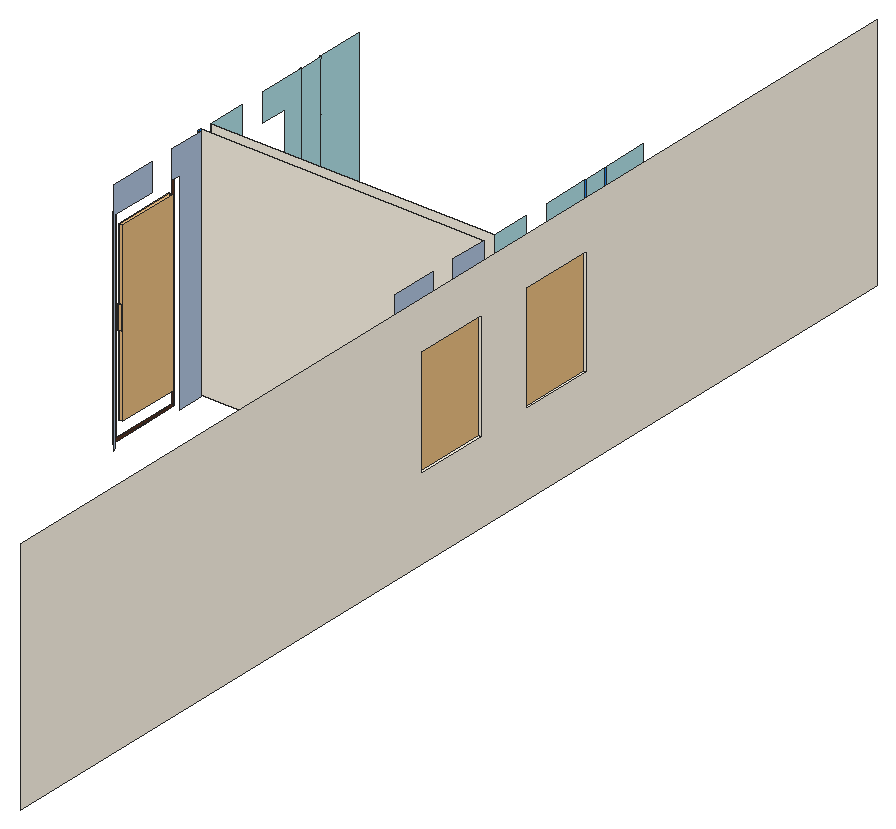
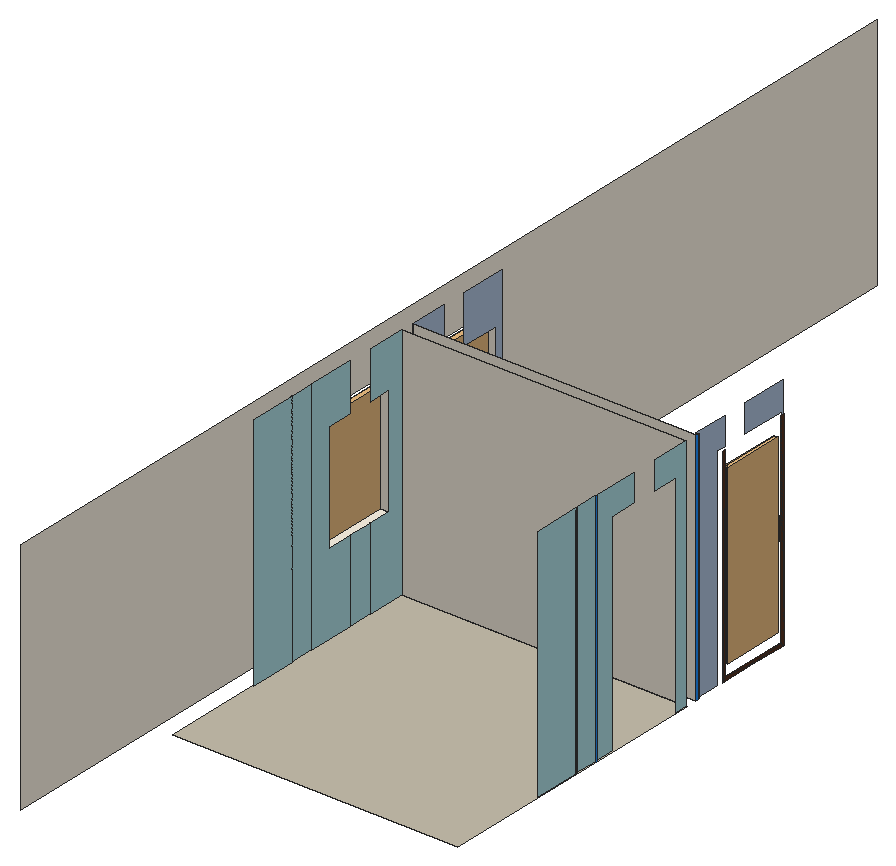
# SketchUp Ruby script. Lengths in inches.
U = 1.inch
M = Sketchup.active_model
def pt(a) = Geom::Point3d.new(a.map { |v| v * U })
def face(e, loops, mat)
  f = e.add_face(loops[0].map { |a| pt(a) })
  loops[1..].each { |l| e.add_face(l.map { |a| pt(a) }).erase! }
  f.material = f.back_material = mat if mat
  f
end
# faces: each face lists its corners as indices into pts; further lists are holes
def faces(e, pts, list, mat = nil) = list.each { |f| face(e, (f[0].is_a?(Array) ? f : [f]).map { |l| l.map { |i| pts[i] } }, mat) }
# xy, xz, yz: faces in a plane at the given z, y or x. An outline is a flat list of corners, or four numbers for a rectangle; further outlines are holes
def ring(l) = l.size == 4 ? [[l[0], l[1]], [l[2], l[1]], [l[2], l[3]], [l[0], l[3]]] : l.each_slice(2).to_a
def flat(e, list, mat, &to3) = list.each { |f| face(e, (f[0].is_a?(Array) ? f : [f]).map { |l| ring(l).map { |u, v| to3.(u, v) } }, mat) }
def xy(e, z, list, mat = nil) = flat(e, list, mat) { |x, y| [x, y, z] }
def xz(e, y, list, mat = nil) = flat(e, list, mat) { |x, z| [x, y, z] }
def yz(e, x, list, mat = nil) = flat(e, list, mat) { |y, z| [x, y, z] }
def lines(e, pts, list) = list.each { |a, b| e.add_line(pt(pts[a]), pt(pts[b])) }
# prism: a flat outline (further loops are holes) pulled along v
def prism(e, loops, v, mat = nil)
  f = face(e, loops, mat); d = Geom::Vector3d.new(v.map { |x| x * U })
  f.pushpull(f.normal.samedirection?(d) ? d.length : -d.length)
end
def box(e, o, s, mat = nil) = prism(e, [[o, [o[0] + s[0], o[1], o[2]], [o[0] + s[0], o[1] + s[1], o[2]], [o[0], o[1] + s[1], o[2]]]], [0, 0, s[2]], mat)
def at(x, y, z, deg = 0) = Geom::Transformation.translation(pt([x, y, z])) * Geom::Transformation.rotation(ORIGIN, Z_AXIS, deg.degrees)
def axes(o, x, y, z) = Geom::Transformation.new([*x, 0, *y, 0, *z, 0, *pt(o).to_a, 1])
def part(name) = M.definitions.add(name)
# library, detail: a bought-in or finely detailed component or shape, given as its bounding box
def library(name, o, s) = part(name).tap { |d| box(d.entities, o, s) }
def detail(e, o, s) = box(e.add_group.entities, o, s)
def put(e, d, t, mat = nil) = e.add_instance(d, t).tap { |i| i.material = mat if mat }
def group(e, t, mat = nil) = e.add_group.tap { |g| g.transformation = t; g.material = mat if mat }.entities
root = M.entities
M.materials.add("Material \#0").color = [86, 53, 35]
M.materials.add("Material \#1").color = [140, 140, 140]
M.materials.add("[0030_OldLace]").color = [253, 245, 230]
M.materials.add("[0094_PowderBlue]").color = [176, 224, 230]
M.materials.add("[0098_DodgerBlue]").color = [30, 144, 255]
M.materials.add("[0099_LightSteelBlue]").color = [176, 196, 222]
M.materials.add("[Tile Canvas]").color = [199, 192, 173]
c1 = library("3DGeom~4_Defintion",[-18.02,-499.97,-221.16],[36.04,1000,262.12])
c2 = part("3DGeom~5_Defintion")
xy(c2.entities,-225.24,[[-0.79,-499.98,-2.33,-499.64,7.45,-496.14],[-0.79,-499.98,7.45,-496.14,1.58,-499.88],[1.58,-499.88,7.45,-496.14,3.84,-499.16],[-2.33,-499.64,7.4,-485.75,7.45,-496.14],[3.84,-499.16,7.45,-496.14,5.85,-497.89],
  [7.45,-496.14,7.4,-485.75,8.24,-487.08],[7.45,-496.14,8.24,-487.08,8.96,-489.34],[7.45,-496.14,8.96,-489.34,9.0625,-491.71],[7.45,-496.14,9.0625,-491.71,8.55,-494.03],[-7.4,-496.08,-8.24,-494.76,2.32,-482.2],
  [-8.24,-494.76,-8.96,-492.5,2.32,-482.2],[-8.96,-492.5,-9.0625,-490.125,2.32,-482.2],[-9.0625,-490.125,-8.55,-487.81,2.32,-482.2],[-8.55,-487.81,-7.45,-485.7,2.32,-482.2],[-7.45,-485.7,-5.85,-483.95,2.32,-482.2],
  [-5.85,-483.95,-3.84,-482.68,2.32,-482.2],[-3.84,-482.68,-1.58,-481.96,2.32,-482.2],[2.32,-482.2,-1.58,-481.96,0.79,-481.86],[0,481.82,-2.35,482.13,-6.92,496.71],[0,481.82,-6.92,496.71,1.55,482.04],
  [-2.35,482.13,-4.55,483.04,-6.92,496.71],[-4.55,483.04,-6.43,484.49,-6.92,496.71],[-6.43,484.49,-7.88,486.37,-6.92,496.71],[6.92,485.12,-1.55,499.8125,7.88,495.47],[6.92,485.12,7.88,495.47,7.88,486.37],
  [-7.88,486.37,-8.79,488.57,-6.92,496.71],[7.88,486.37,7.88,495.47,8.79,488.57],[-8.79,488.57,-9.1,490.92,-6.92,496.71],[8.79,488.57,7.88,495.47,9.1,490.92],[-9.1,490.92,-8.79,493.28,-6.92,496.71],
  [9.1,490.92,7.88,495.47,8.79,493.28],[-8.79,493.28,-7.88,495.47,-6.92,496.71],[7.88,495.47,-1.55,499.8125,0,500.02],[7.88,495.47,0,500.02,2.35,499.71],[7.88,495.47,2.35,499.71,4.55,498.8],
  [7.88,495.47,4.55,498.8,6.43,497.35]],"Material \#1")
xy(c2.entities,-221.57,[[-2.33,-499.64,-5.22,-498.37,7.4,-485.75],[-5.22,-498.37,-7.4,-496.08,5.22,-483.47],[-5.22,-498.37,5.22,-483.47,7.4,-485.75],[-7.4,-496.08,2.32,-482.2,5.22,-483.47],[1.55,482.04,-6.92,496.71,-4.55,498.8],
  [1.55,482.04,-4.55,498.8,4.55,483.04],[4.55,483.04,-4.55,498.8,-1.55,499.8125],[4.55,483.04,-1.55,499.8125,6.92,485.12]],"Material \#1")
xy(c2.entities,38.05,[[-2.33,-499.64,7.4,-485.75,-5.22,-498.37],[-5.22,-498.37,5.22,-483.47,-7.4,-496.08],[-5.22,-498.37,7.4,-485.75,5.22,-483.47],[-7.4,-496.08,5.22,-483.47,2.32,-482.2],[1.55,482.04,-4.55,498.8,-6.92,496.71],
  [1.55,482.04,4.55,483.04,-4.55,498.8],[4.55,483.04,-1.55,499.8125,-4.55,498.8],[4.55,483.04,6.92,485.12,-1.55,499.8125]],"Material \#1")
xy(c2.entities,41.72,[[-0.79,-499.98,7.45,-496.14,-2.33,-499.64],[-0.79,-499.98,1.58,-499.88,7.45,-496.14],[1.58,-499.88,3.84,-499.16,7.45,-496.14],[-2.33,-499.64,7.45,-496.14,7.4,-485.75],[3.84,-499.16,5.85,-497.89,7.45,-496.14],
  [7.45,-496.14,8.24,-487.08,7.4,-485.75],[7.45,-496.14,8.55,-494.03,9.0625,-491.71],[7.45,-496.14,8.96,-489.34,8.24,-487.08],[7.45,-496.14,9.0625,-491.71,8.96,-489.34],[-7.4,-496.08,2.32,-482.2,-8.24,-494.76],
  [-8.24,-494.76,2.32,-482.2,-8.96,-492.5],[-8.96,-492.5,2.32,-482.2,-9.0625,-490.125],[-9.0625,-490.125,2.32,-482.2,-8.55,-487.81],[-8.55,-487.81,2.32,-482.2,-7.45,-485.7],[-7.45,-485.7,2.32,-482.2,-5.85,-483.95],
  [-5.85,-483.95,2.32,-482.2,-3.84,-482.68],[-3.84,-482.68,2.32,-482.2,-1.58,-481.96],[2.32,-482.2,0.79,-481.86,-1.58,-481.96],[0,481.82,-6.92,496.71,-2.35,482.13],[0,481.82,1.55,482.04,-6.92,496.71],
  [-2.35,482.13,-6.92,496.71,-4.55,483.04],[-4.55,483.04,-6.92,496.71,-6.43,484.49],[-6.43,484.49,-6.92,496.71,-7.88,486.37],[6.92,485.12,7.88,495.47,-1.55,499.8125],[6.92,485.12,7.88,486.37,7.88,495.47],
  [-7.88,486.37,-6.92,496.71,-8.79,488.57],[7.88,486.37,8.79,488.57,7.88,495.47],[-8.79,488.57,-6.92,496.71,-9.1,490.92],[8.79,488.57,9.1,490.92,7.88,495.47],[-9.1,490.92,-6.92,496.71,-8.79,493.28],
  [9.1,490.92,8.79,493.28,7.88,495.47],[-8.79,493.28,-6.92,496.71,-7.88,495.47],[7.88,495.47,0,500.02,-1.55,499.8125],[7.88,495.47,2.35,499.71,0,500.02],[7.88,495.47,4.55,498.8,2.35,499.71],
  [7.88,495.47,6.43,497.35,4.55,498.8]],"Material \#1")
c3 = library("3DGeom~14_Defintion",[-102.17,352.37,-727.27],[204.35,204.35,1000])
c4 = library("3DGeom~1_Defintion",[-60.87,347.29,-704.08],[121.74,121.75,1000])
c5 = library("3DGeom~3_Defintion",[-83.33,-500,-350],[620.1,1000,533.33])
c6 = part("3DGeom~21_Defintion")
xy(c6.entities,73.08,[[-976.3,-241.71,23.7,-241.71,-976.3,-223.46],[23.7,-241.71,5.45,-223.46,-976.3,-223.46],[23.7,-241.71,23.7,0,5.45,-223.46],[5.45,-223.46,23.7,0,5.45,0],[23.7,0,23.7,241.71,5.45,223.46],
  [5.45,0,23.7,0,5.45,223.46],[-976.3,223.46,23.7,241.71,-976.3,241.71],[-976.3,223.46,5.45,223.46,23.7,241.71]],"Material \#0")
c7 = library("3DGeom~6_Defintion",[-5.59,-471.8,-48.03],[468.87,1000,73.72])
c8 = library("Window 82-25",[-14.97,-2.34,0.01],[29.93,4.71,56.48])
c9 = library("3DGeom~9_Defintion",[456.52,-471.89,-18.89],[5.57,1000,5.49])
c10 = part("3DGeom~8_Defintion")
xz(c10.entities,-471.94,[[458.125,-17.29,459.53,-16.11,457.73,-17.15],[458.125,-17.29,458.54,-17.29,459.53,-16.11],[458.54,-17.29,458.93,-17.15,459.53,-16.11],[457.73,-17.15,459.53,-16.11,457.42,-16.88],[458.93,-17.15,459.25,-16.88,459.53,-16.11],
  [457.42,-16.88,459.53,-16.11,457.21,-16.52],[459.25,-16.88,459.46,-16.52,459.53,-16.11],[457.21,-16.52,459.53,-16.11,457.14,-16.11],[457.14,-16.11,459.53,-16.11,457.21,-15.7],[459.53,-16.11,457.42,-15.34,457.21,-15.7],
  [459.53,-16.11,457.73,-15.07,457.42,-15.34],[459.53,-16.11,458.125,-14.93,457.73,-15.07],[459.53,-16.11,458.54,-14.93,458.125,-14.93],[459.53,-16.11,458.93,-15.07,458.54,-14.93],[459.53,-16.11,459.25,-15.34,458.93,-15.07],
  [459.53,-16.11,459.46,-15.7,459.25,-15.34]],"Material \#1")
xz(c10.entities,-416.39,[[458.125,-17.29,457.73,-17.15,459.53,-16.11],[458.125,-17.29,459.53,-16.11,458.54,-17.29],[458.54,-17.29,459.53,-16.11,458.93,-17.15],[457.73,-17.15,457.42,-16.88,459.53,-16.11],[458.93,-17.15,459.53,-16.11,459.25,-16.88],
  [457.42,-16.88,457.21,-16.52,459.53,-16.11],[459.25,-16.88,459.53,-16.11,459.46,-16.52],[457.21,-16.52,457.14,-16.11,459.53,-16.11],[457.14,-16.11,457.21,-15.7,459.53,-16.11],[459.53,-16.11,457.21,-15.7,457.42,-15.34],
  [459.53,-16.11,457.42,-15.34,457.73,-15.07],[459.53,-16.11,457.73,-15.07,458.125,-14.93],[459.53,-16.11,458.125,-14.93,458.54,-14.93],[459.53,-16.11,458.54,-14.93,458.93,-15.07],[459.53,-16.11,458.93,-15.07,459.25,-15.34],
  [459.53,-16.11,459.25,-15.34,459.46,-15.7]],"Material \#1")
xz(c10.entities,-27.5,[[458.125,-17.29,459.53,-16.11,457.73,-17.15],[458.125,-17.29,458.54,-17.29,459.53,-16.11],[458.54,-17.29,458.93,-17.15,459.53,-16.11],[457.73,-17.15,459.53,-16.11,457.42,-16.88],[458.93,-17.15,459.25,-16.88,459.53,-16.11],
  [457.42,-16.88,459.53,-16.11,457.21,-16.52],[459.25,-16.88,459.46,-16.52,459.53,-16.11],[457.21,-16.52,459.53,-16.11,457.14,-16.11],[457.14,-16.11,459.53,-16.11,457.21,-15.7],[459.53,-16.11,457.42,-15.34,457.21,-15.7],
  [459.53,-16.11,457.73,-15.07,457.42,-15.34],[459.53,-16.11,458.125,-14.93,457.73,-15.07],[459.53,-16.11,458.54,-14.93,458.125,-14.93],[459.53,-16.11,458.93,-15.07,458.54,-14.93],[459.53,-16.11,459.25,-15.34,458.93,-15.07],
  [459.53,-16.11,459.46,-15.7,459.25,-15.34]],"Material \#1")
xz(c10.entities,28.06,[[458.125,-17.29,457.73,-17.15,459.53,-16.11],[458.125,-17.29,459.53,-16.11,458.54,-17.29],[458.54,-17.29,459.53,-16.11,458.93,-17.15],[457.73,-17.15,457.42,-16.88,459.53,-16.11],[458.93,-17.15,459.53,-16.11,459.25,-16.88],
  [457.42,-16.88,457.21,-16.52,459.53,-16.11],[459.25,-16.88,459.53,-16.11,459.46,-16.52],[457.21,-16.52,457.14,-16.11,459.53,-16.11],[457.14,-16.11,457.21,-15.7,459.53,-16.11],[459.53,-16.11,457.21,-15.7,457.42,-15.34],
  [459.53,-16.11,457.42,-15.34,457.73,-15.07],[459.53,-16.11,457.73,-15.07,458.125,-14.93],[459.53,-16.11,458.125,-14.93,458.54,-14.93],[459.53,-16.11,458.54,-14.93,458.93,-15.07],[459.53,-16.11,458.93,-15.07,459.25,-15.34],
  [459.53,-16.11,459.25,-15.34,459.46,-15.7]],"Material \#1")
xz(c10.entities,472.5,[[458.125,-17.29,459.53,-16.11,457.73,-17.15],[458.125,-17.29,458.54,-17.29,459.53,-16.11],[458.54,-17.29,458.93,-17.15,459.53,-16.11],[457.73,-17.15,459.53,-16.11,457.42,-16.88],[458.93,-17.15,459.25,-16.88,459.53,-16.11],
  [457.42,-16.88,459.53,-16.11,457.21,-16.52],[459.25,-16.88,459.46,-16.52,459.53,-16.11],[457.21,-16.52,459.53,-16.11,457.14,-16.11],[457.14,-16.11,459.53,-16.11,457.21,-15.7],[459.53,-16.11,457.42,-15.34,457.21,-15.7],
  [459.53,-16.11,457.73,-15.07,457.42,-15.34],[459.53,-16.11,458.125,-14.93,457.73,-15.07],[459.53,-16.11,458.54,-14.93,458.125,-14.93],[459.53,-16.11,458.93,-15.07,458.54,-14.93],[459.53,-16.11,459.25,-15.34,458.93,-15.07],
  [459.53,-16.11,459.46,-15.7,459.25,-15.34]],"Material \#1")
xz(c10.entities,528.06,[[458.125,-17.29,457.73,-17.15,459.53,-16.11],[458.125,-17.29,459.53,-16.11,458.54,-17.29],[458.54,-17.29,459.53,-16.11,458.93,-17.15],[457.73,-17.15,457.42,-16.88,459.53,-16.11],[458.93,-17.15,459.53,-16.11,459.25,-16.88],
  [457.42,-16.88,457.21,-16.52,459.53,-16.11],[459.25,-16.88,459.53,-16.11,459.46,-16.52],[457.21,-16.52,457.14,-16.11,459.53,-16.11],[457.14,-16.11,457.21,-15.7,459.53,-16.11],[459.53,-16.11,457.21,-15.7,457.42,-15.34],
  [459.53,-16.11,457.42,-15.34,457.73,-15.07],[459.53,-16.11,457.73,-15.07,458.125,-14.93],[459.53,-16.11,458.125,-14.93,458.54,-14.93],[459.53,-16.11,458.54,-14.93,458.93,-15.07],[459.53,-16.11,458.93,-15.07,459.25,-15.34],
  [459.53,-16.11,459.25,-15.34,459.46,-15.7]],"Material \#1")
c11 = library("3DGeom~7_Defintion",[455.56,-471.94,-18.85],[5.55,1000,5.48])
xy(root,9.622,[[266.181,291.258,266.159,291.287,266.157,291.269],[266.181,291.258,266.181,291.277,266.159,291.287],[266.181,291.258,266.205,291.269,266.181,291.277],[266.157,291.269,266.14,291.316,266.135,291.302],[266.157,291.269,266.159,291.287,266.14,291.316],
  [266.205,291.269,266.203,291.287,266.181,291.277],[266.205,291.269,266.227,291.302,266.203,291.287],[266.203,291.287,266.227,291.302,266.222,291.316],[266.135,291.302,266.126,291.361,266.12,291.352],[266.135,291.302,266.14,291.316,266.126,291.361],
  [266.227,291.302,266.243,291.352,266.222,291.316],[266.222,291.316,266.243,291.352,266.237,291.361],[266.12,291.352,266.118,291.416,266.111,291.413],[266.12,291.352,266.126,291.361,266.118,291.416],[266.243,291.352,266.251,291.413,266.237,291.361],
  [266.237,291.361,266.251,291.413,266.244,291.416],[266.111,291.413,266.118,291.416,266.118,291.475],[266.111,291.413,266.118,291.475,266.111,291.478],[266.251,291.413,266.251,291.478,266.244,291.416],[266.244,291.416,266.251,291.478,266.244,291.475],
  [266.118,291.475,266.126,291.53,266.111,291.478],[266.244,291.475,266.243,291.539,266.237,291.53],[266.244,291.475,266.251,291.478,266.243,291.539],[266.111,291.478,266.126,291.53,266.12,291.539],[266.126,291.53,266.14,291.574,266.12,291.539],
  [266.237,291.53,266.227,291.589,266.222,291.574],[266.237,291.53,266.243,291.539,266.227,291.589],[266.12,291.539,266.14,291.574,266.135,291.589],[266.14,291.574,266.159,291.604,266.135,291.589],[266.222,291.574,266.205,291.621,266.203,291.604],
  [266.222,291.574,266.227,291.589,266.205,291.621],[266.135,291.589,266.159,291.604,266.157,291.621],[266.159,291.604,266.181,291.614,266.157,291.621],[266.203,291.604,266.181,291.633,266.181,291.614],[266.203,291.604,266.205,291.621,266.181,291.633],
  [266.181,291.614,266.181,291.633,266.157,291.621]],"Material \#1")
xy(root,9.642,[[266.181,291.258,266.157,291.269,266.181,291.277],[266.181,291.258,266.181,291.277,266.203,291.287],[266.181,291.258,266.203,291.287,266.205,291.269],[266.157,291.269,266.135,291.302,266.159,291.287],[266.157,291.269,266.159,291.287,266.181,291.277],
  [266.205,291.269,266.203,291.287,266.222,291.316],[266.205,291.269,266.222,291.316,266.227,291.302],[266.159,291.287,266.135,291.302,266.14,291.316],[266.135,291.302,266.12,291.352,266.14,291.316],[266.227,291.302,266.222,291.316,266.237,291.361],
  [266.227,291.302,266.237,291.361,266.243,291.352],[266.14,291.316,266.12,291.352,266.126,291.361],[266.12,291.352,266.111,291.413,266.126,291.361],[266.243,291.352,266.237,291.361,266.244,291.416],[266.243,291.352,266.244,291.416,266.251,291.413],
  [266.126,291.361,266.111,291.413,266.118,291.416],[266.111,291.413,266.111,291.478,266.118,291.416],[266.251,291.413,266.244,291.416,266.244,291.475],[266.251,291.413,266.244,291.475,266.251,291.478],[266.118,291.416,266.111,291.478,266.118,291.475],
  [266.118,291.475,266.111,291.478,266.12,291.539],[266.118,291.475,266.12,291.539,266.126,291.53],[266.244,291.475,266.237,291.53,266.251,291.478],[266.251,291.478,266.237,291.53,266.243,291.539],[266.126,291.53,266.12,291.539,266.135,291.589],
  [266.126,291.53,266.135,291.589,266.14,291.574],[266.237,291.53,266.222,291.574,266.243,291.539],[266.243,291.539,266.222,291.574,266.227,291.589],[266.14,291.574,266.135,291.589,266.157,291.621],[266.14,291.574,266.157,291.621,266.159,291.604],
  [266.222,291.574,266.203,291.604,266.227,291.589],[266.227,291.589,266.203,291.604,266.205,291.621],[266.159,291.604,266.157,291.621,266.181,291.633],[266.159,291.604,266.181,291.633,266.181,291.614],[266.203,291.604,266.181,291.614,266.205,291.621],
  [266.181,291.614,266.181,291.633,266.205,291.621]],"Material \#1")
xy(root,14.085,[[266.181,291.258,266.181,291.277,266.157,291.269],[266.181,291.258,266.203,291.287,266.181,291.277],[266.181,291.258,266.205,291.269,266.203,291.287],[266.157,291.269,266.159,291.287,266.135,291.302],[266.157,291.269,266.181,291.277,266.159,291.287],
  [266.205,291.269,266.222,291.316,266.203,291.287],[266.205,291.269,266.227,291.302,266.222,291.316],[266.159,291.287,266.14,291.316,266.135,291.302],[266.135,291.302,266.14,291.316,266.12,291.352],[266.227,291.302,266.237,291.361,266.222,291.316],
  [266.227,291.302,266.243,291.352,266.237,291.361],[266.14,291.316,266.126,291.361,266.12,291.352],[266.12,291.352,266.126,291.361,266.111,291.413],[266.243,291.352,266.244,291.416,266.237,291.361],[266.243,291.352,266.251,291.413,266.244,291.416],
  [266.126,291.361,266.118,291.416,266.111,291.413],[266.111,291.413,266.118,291.416,266.111,291.478],[266.251,291.413,266.244,291.475,266.244,291.416],[266.251,291.413,266.251,291.478,266.244,291.475],[266.118,291.416,266.118,291.475,266.111,291.478],
  [266.118,291.475,266.12,291.539,266.111,291.478],[266.118,291.475,266.126,291.53,266.12,291.539],[266.244,291.475,266.251,291.478,266.237,291.53],[266.251,291.478,266.243,291.539,266.237,291.53],[266.126,291.53,266.135,291.589,266.12,291.539],
  [266.126,291.53,266.14,291.574,266.135,291.589],[266.237,291.53,266.243,291.539,266.222,291.574],[266.243,291.539,266.227,291.589,266.222,291.574],[266.14,291.574,266.157,291.621,266.135,291.589],[266.14,291.574,266.159,291.604,266.157,291.621],
  [266.222,291.574,266.227,291.589,266.203,291.604],[266.227,291.589,266.205,291.621,266.203,291.604],[266.159,291.604,266.181,291.633,266.157,291.621],[266.159,291.604,266.181,291.614,266.181,291.633],[266.203,291.604,266.205,291.621,266.181,291.614],
  [266.181,291.614,266.205,291.621,266.181,291.633]],"Material \#1")
xy(root,14.104,[[266.181,291.258,266.157,291.269,266.159,291.287],[266.181,291.258,266.159,291.287,266.181,291.277],[266.181,291.258,266.181,291.277,266.205,291.269],[266.157,291.269,266.135,291.302,266.14,291.316],[266.157,291.269,266.14,291.316,266.159,291.287],
  [266.205,291.269,266.181,291.277,266.203,291.287],[266.205,291.269,266.203,291.287,266.227,291.302],[266.203,291.287,266.222,291.316,266.227,291.302],[266.135,291.302,266.12,291.352,266.126,291.361],[266.135,291.302,266.126,291.361,266.14,291.316],
  [266.227,291.302,266.222,291.316,266.243,291.352],[266.222,291.316,266.237,291.361,266.243,291.352],[266.12,291.352,266.111,291.413,266.118,291.416],[266.12,291.352,266.118,291.416,266.126,291.361],[266.243,291.352,266.237,291.361,266.251,291.413],
  [266.237,291.361,266.244,291.416,266.251,291.413],[266.111,291.413,266.111,291.478,266.118,291.475],[266.111,291.413,266.118,291.475,266.118,291.416],[266.251,291.413,266.244,291.416,266.251,291.478],[266.244,291.416,266.244,291.475,266.251,291.478],
  [266.118,291.475,266.111,291.478,266.126,291.53],[266.244,291.475,266.237,291.53,266.243,291.539],[266.244,291.475,266.243,291.539,266.251,291.478],[266.111,291.478,266.12,291.539,266.126,291.53],[266.126,291.53,266.12,291.539,266.14,291.574],
  [266.237,291.53,266.222,291.574,266.227,291.589],[266.237,291.53,266.227,291.589,266.243,291.539],[266.12,291.539,266.135,291.589,266.14,291.574],[266.14,291.574,266.135,291.589,266.159,291.604],[266.222,291.574,266.203,291.604,266.205,291.621],
  [266.222,291.574,266.205,291.621,266.227,291.589],[266.135,291.589,266.157,291.621,266.159,291.604],[266.159,291.604,266.157,291.621,266.181,291.614],[266.203,291.604,266.181,291.614,266.181,291.633],[266.203,291.604,266.181,291.633,266.205,291.621],
  [266.181,291.614,266.157,291.621,266.181,291.633]],"Material \#1")
xy(root,41,[[410,257.09,420,257.09,420,295.465,410,295.465,410,289.965,411,289.965,411,289.465,410,289.465,410,277.465,411,277.465,411,276.965,410,276.965],[410.75,323.465,420,323.465,420,361.527,410.75,361.527,410.75,347.965,411,347.965,411,347.465,410.75,347.465,410.75,335.465,411,335.465,411,334.965,410.75,334.965]],"[0030_OldLace]")
xy(root,54.201,[[266.181,291.258,266.159,291.287,266.157,291.269],[266.181,291.258,266.181,291.277,266.159,291.287],[266.181,291.258,266.205,291.269,266.181,291.277],[266.157,291.269,266.14,291.316,266.135,291.302],[266.157,291.269,266.159,291.287,266.14,291.316],
  [266.205,291.269,266.203,291.287,266.181,291.277],[266.205,291.269,266.227,291.302,266.203,291.287],[266.203,291.287,266.227,291.302,266.222,291.316],[266.135,291.302,266.126,291.361,266.12,291.352],[266.135,291.302,266.14,291.316,266.126,291.361],
  [266.227,291.302,266.243,291.352,266.222,291.316],[266.222,291.316,266.243,291.352,266.237,291.361],[266.12,291.352,266.118,291.416,266.111,291.413],[266.12,291.352,266.126,291.361,266.118,291.416],[266.243,291.352,266.251,291.413,266.237,291.361],
  [266.237,291.361,266.251,291.413,266.244,291.416],[266.111,291.413,266.118,291.416,266.118,291.475],[266.111,291.413,266.118,291.475,266.111,291.478],[266.251,291.413,266.251,291.478,266.244,291.416],[266.244,291.416,266.251,291.478,266.244,291.475],
  [266.118,291.475,266.126,291.53,266.111,291.478],[266.244,291.475,266.243,291.539,266.237,291.53],[266.244,291.475,266.251,291.478,266.243,291.539],[266.111,291.478,266.126,291.53,266.12,291.539],[266.126,291.53,266.14,291.574,266.12,291.539],
  [266.237,291.53,266.227,291.589,266.222,291.574],[266.237,291.53,266.243,291.539,266.227,291.589],[266.12,291.539,266.14,291.574,266.135,291.589],[266.14,291.574,266.159,291.604,266.135,291.589],[266.222,291.574,266.205,291.621,266.203,291.604],
  [266.222,291.574,266.227,291.589,266.205,291.621],[266.135,291.589,266.159,291.604,266.157,291.621],[266.159,291.604,266.181,291.614,266.157,291.621],[266.203,291.604,266.181,291.633,266.181,291.614],[266.203,291.604,266.205,291.621,266.181,291.633],
  [266.181,291.614,266.181,291.633,266.157,291.621]],"Material \#1")
xy(root,54.221,[[266.181,291.258,266.157,291.269,266.181,291.277],[266.181,291.258,266.181,291.277,266.203,291.287],[266.181,291.258,266.203,291.287,266.205,291.269],[266.157,291.269,266.135,291.302,266.159,291.287],[266.157,291.269,266.159,291.287,266.181,291.277],
  [266.205,291.269,266.203,291.287,266.222,291.316],[266.205,291.269,266.222,291.316,266.227,291.302],[266.159,291.287,266.135,291.302,266.14,291.316],[266.135,291.302,266.12,291.352,266.14,291.316],[266.227,291.302,266.222,291.316,266.237,291.361],
  [266.227,291.302,266.237,291.361,266.243,291.352],[266.14,291.316,266.12,291.352,266.126,291.361],[266.12,291.352,266.111,291.413,266.126,291.361],[266.243,291.352,266.237,291.361,266.244,291.416],[266.243,291.352,266.244,291.416,266.251,291.413],
  [266.126,291.361,266.111,291.413,266.118,291.416],[266.111,291.413,266.111,291.478,266.118,291.416],[266.251,291.413,266.244,291.416,266.244,291.475],[266.251,291.413,266.244,291.475,266.251,291.478],[266.118,291.416,266.111,291.478,266.118,291.475],
  [266.118,291.475,266.111,291.478,266.12,291.539],[266.118,291.475,266.12,291.539,266.126,291.53],[266.244,291.475,266.237,291.53,266.251,291.478],[266.251,291.478,266.237,291.53,266.243,291.539],[266.126,291.53,266.12,291.539,266.135,291.589],
  [266.126,291.53,266.135,291.589,266.14,291.574],[266.237,291.53,266.222,291.574,266.243,291.539],[266.243,291.539,266.222,291.574,266.227,291.589],[266.14,291.574,266.135,291.589,266.157,291.621],[266.14,291.574,266.157,291.621,266.159,291.604],
  [266.222,291.574,266.203,291.604,266.227,291.589],[266.227,291.589,266.203,291.604,266.205,291.621],[266.159,291.604,266.157,291.621,266.181,291.633],[266.159,291.604,266.181,291.633,266.181,291.614],[266.203,291.604,266.181,291.614,266.205,291.621],
  [266.181,291.614,266.181,291.633,266.205,291.621]],"Material \#1")
xz(root,276.965,[[410,0,411,41]],"[0098_DodgerBlue]")
xz(root,277.465,[[410,0,411,41]],"[0098_DodgerBlue]")
xz(root,289.465,[[410,0,411,41]],"[0098_DodgerBlue]")
xz(root,289.965,[[410,0,411,41]],"[0098_DodgerBlue]")
xz(root,295.465,[[410,41,420,96]],"[0030_OldLace]")
xz(root,307.965,[[267,0,268.125,120]],"[0030_OldLace]")
xz(root,309.465,[[267,0,410,120]],"[0030_OldLace]")
xz(root,315.465,[[267.4375,0,410.75,120]],"[0030_OldLace]")
xz(root,323.465,[[410.75,41,420,96]],"[0030_OldLace]")
xz(root,334.965,[[410.75,0,411,41]],"[0098_DodgerBlue]")
xz(root,335.465,[[410.75,0,411,41]],"[0098_DodgerBlue]")
xz(root,347.465,[[410.75,0,411,41]],"[0098_DodgerBlue]")
xz(root,347.965,[[410.75,0,411,41]],"[0098_DodgerBlue]")
xz(root,361.527,[[410.75,41,420,96]],"[0030_OldLace]")
xz(root,371.959,[[267,0,267.4375,120]],"[0098_DodgerBlue]")
xz(root,371.965,[[410.75,0,411,120]],"[0098_DodgerBlue]")
xz(root,372.465,[[410.75,0,411,120]],"[0098_DodgerBlue]")
xz(root,372.47,[[267,0,267.4375,120]],"[0098_DodgerBlue]")
xz(root,384.441,[[267,0,267.4375,120]],"[0098_DodgerBlue]")
xz(root,384.458,[[410.75,0,411,120]],"[0098_DodgerBlue]")
xz(root,384.939,[[267,0,267.4375,120]],"[0098_DodgerBlue]")
xz(root,384.961,[[410.75,0,411,120]],"[0098_DodgerBlue]")
yz(root,265.641,[[260.515,50.648,260.399,50.676,260.515,50.663],[260.515,50.648,260.515,50.663,260.633,50.662],[260.633,50.662,260.515,50.663,260.631,50.676],[260.633,50.662,260.631,50.676,260.743,50.702],[260.631,50.676,260.74,50.716,260.743,50.702],
  [260.743,50.702,260.74,50.716,260.846,50.766],[260.74,50.716,260.84,50.779,260.846,50.766],[260.846,50.766,260.84,50.779,260.937,50.852],[260.84,50.779,260.93,50.863,260.937,50.852],[260.937,50.852,260.93,50.863,261.016,50.956],
  [260.93,50.863,261.008,50.966,261.016,50.956],[260.515,50.879,260.476,50.884,260.478,50.899],[260.515,50.879,260.478,50.899,260.515,50.894],[260.515,50.879,260.515,50.894,260.554,50.884],[260.554,50.884,260.515,50.894,260.552,50.899],
  [260.554,50.884,260.552,50.899,260.591,50.898],[260.591,50.898,260.552,50.899,260.587,50.911],[260.591,50.898,260.587,50.911,260.625,50.919],[260.587,50.911,260.619,50.932,260.625,50.919],[260.625,50.919,260.619,50.932,260.655,50.947],
  [260.619,50.932,260.648,50.959,260.655,50.947],[260.655,50.947,260.648,50.959,260.681,50.982],[261.016,50.956,261.008,50.966,261.081,51.077],[260.648,50.959,260.673,50.991,260.681,50.982],[261.008,50.966,261.071,51.085,261.081,51.077],
  [260.681,50.982,260.673,50.991,260.703,51.022],[260.673,50.991,260.693,51.03,260.703,51.022],[260.703,51.022,260.693,51.03,260.719,51.067],[260.693,51.03,260.708,51.072,260.719,51.067],[260.719,51.067,260.708,51.072,260.729,51.116],
  [260.708,51.072,260.718,51.118,260.729,51.116],[261.081,51.077,261.071,51.085,261.129,51.212],[261.071,51.085,261.119,51.217,261.129,51.212],[260.729,51.116,260.718,51.118,260.733,51.167],[260.718,51.118,260.721,51.167,260.733,51.167],
  [260.721,51.167,260.718,51.216,260.729,51.219],[260.721,51.167,260.729,51.219,260.733,51.167],[261.129,51.212,261.119,51.217,261.16,51.358],[260.718,51.216,260.708,51.262,260.719,51.268],[260.718,51.216,260.719,51.268,260.729,51.219],
  [261.119,51.217,261.149,51.361,261.16,51.358],[260.708,51.262,260.693,51.305,260.703,51.3125],[260.708,51.262,260.703,51.3125,260.719,51.268],[260.693,51.305,260.673,51.343,260.681,51.353],[260.693,51.305,260.681,51.353,260.703,51.3125],
  [260.673,51.343,260.648,51.376,260.655,51.387],[260.673,51.343,260.655,51.387,260.681,51.353],[261.16,51.358,261.149,51.361,261.171,51.52],[261.149,51.361,261.16,51.52,261.171,51.52],[260.648,51.376,260.619,51.403,260.625,51.416],
  [260.648,51.376,260.625,51.416,260.655,51.387],[260.619,51.403,260.587,51.423,260.591,51.437],[260.619,51.403,260.591,51.437,260.625,51.416],[260.587,51.423,260.552,51.436,260.554,51.451],[260.587,51.423,260.554,51.451,260.591,51.437],
  [260.478,51.436,260.476,51.451,260.515,51.44],[260.552,51.436,260.515,51.44,260.515,51.455],[260.552,51.436,260.515,51.455,260.554,51.451],[260.515,51.44,260.476,51.451,260.515,51.455],[261.16,51.52,261.16,53.653,261.171,61.415],
  [261.16,51.52,261.171,61.415,261.171,51.52]],"Material \#1")
yz(root,266.465,[[260.515,50.648,260.515,50.663,260.399,50.676],[260.515,50.648,260.633,50.662,260.515,50.663],[260.633,50.662,260.631,50.676,260.515,50.663],[260.633,50.662,260.743,50.702,260.631,50.676],[260.631,50.676,260.743,50.702,260.74,50.716],
  [260.743,50.702,260.846,50.766,260.74,50.716],[260.74,50.716,260.846,50.766,260.84,50.779],[260.846,50.766,260.937,50.852,260.84,50.779],[260.84,50.779,260.937,50.852,260.93,50.863],[260.937,50.852,261.016,50.956,260.93,50.863],
  [260.93,50.863,261.016,50.956,261.008,50.966],[260.515,50.879,260.478,50.899,260.476,50.884],[260.515,50.879,260.515,50.894,260.478,50.899],[260.515,50.879,260.554,50.884,260.515,50.894],[260.554,50.884,260.552,50.899,260.515,50.894],
  [260.554,50.884,260.591,50.898,260.552,50.899],[260.591,50.898,260.587,50.911,260.552,50.899],[260.591,50.898,260.625,50.919,260.587,50.911],[260.587,50.911,260.625,50.919,260.619,50.932],[260.625,50.919,260.655,50.947,260.619,50.932],
  [260.619,50.932,260.655,50.947,260.648,50.959],[260.655,50.947,260.681,50.982,260.648,50.959],[261.016,50.956,261.081,51.077,261.008,50.966],[260.648,50.959,260.681,50.982,260.673,50.991],[261.008,50.966,261.081,51.077,261.071,51.085],
  [260.681,50.982,260.703,51.022,260.673,50.991],[260.673,50.991,260.703,51.022,260.693,51.03],[260.703,51.022,260.719,51.067,260.693,51.03],[260.693,51.03,260.719,51.067,260.708,51.072],[260.719,51.067,260.729,51.116,260.708,51.072],
  [260.708,51.072,260.729,51.116,260.718,51.118],[261.081,51.077,261.129,51.212,261.071,51.085],[261.071,51.085,261.129,51.212,261.119,51.217],[260.729,51.116,260.733,51.167,260.718,51.118],[260.718,51.118,260.733,51.167,260.721,51.167],
  [260.721,51.167,260.729,51.219,260.718,51.216],[260.721,51.167,260.733,51.167,260.729,51.219],[261.129,51.212,261.16,51.358,261.119,51.217],[260.718,51.216,260.719,51.268,260.708,51.262],[260.718,51.216,260.729,51.219,260.719,51.268],
  [261.119,51.217,261.16,51.358,261.149,51.361],[260.708,51.262,260.703,51.3125,260.693,51.305],[260.708,51.262,260.719,51.268,260.703,51.3125],[260.693,51.305,260.681,51.353,260.673,51.343],[260.693,51.305,260.703,51.3125,260.681,51.353],
  [260.673,51.343,260.655,51.387,260.648,51.376],[260.673,51.343,260.681,51.353,260.655,51.387],[261.16,51.358,261.171,51.52,261.149,51.361],[261.149,51.361,261.171,51.52,261.16,51.52],[260.648,51.376,260.625,51.416,260.619,51.403],
  [260.648,51.376,260.655,51.387,260.625,51.416],[260.619,51.403,260.591,51.437,260.587,51.423],[260.619,51.403,260.625,51.416,260.591,51.437],[260.587,51.423,260.554,51.451,260.552,51.436],[260.587,51.423,260.591,51.437,260.554,51.451],
  [260.478,51.436,260.515,51.44,260.476,51.451],[260.552,51.436,260.515,51.455,260.515,51.44],[260.552,51.436,260.554,51.451,260.515,51.455],[260.515,51.44,260.515,51.455,260.476,51.451],[261.16,51.52,261.171,51.52,261.171,61.415],
  [261.16,51.52,261.171,61.415,261.16,53.653],[261.16,53.653,261.171,61.415,261.16,61.414]],"Material \#1")
yz(root,267,[[307.965,0,308.507,120],[308.507,0,309.465,120],[371.959,0,372.47,120],[384.441,0,384.939,120]],"[0098_DodgerBlue]")
yz(root,267.4375,[[315.465,0,321.882,0,321.882,106,334.965,106,334.965,120,315.465,120],[361.777,0,371.959,0,371.959,120,347.965,120,347.965,106,361.777,106],[372.47,0,384.441,120],[384.939,0,408.963,120]],"[0094_PowderBlue]")
yz(root,268.125,[[252.996,0,254.141,0,254.141,106,276.965,106,276.965,120,252.996,120],[294.632,0,307.965,0,307.965,120,289.965,120,289.965,106,294.632,106]],"[0099_LightSteelBlue]")
yz(root,410,[[252.965,0,252.965,120,276.965,120,276.965,96,257.09,96,257.09,41,276.965,41,276.965,0],[277.465,0,289.465,41],[289.965,0,289.965,41,295.465,41,295.465,96,289.965,96,289.965,120,309.465,120,309.465,0]],"[0099_LightSteelBlue]")
yz(root,410.75,[[315.465,0,315.465,120,334.965,120,334.965,96,323.465,96,323.465,41,334.965,41,334.965,0],[335.465,0,347.465,41],[347.965,0,347.965,41,361.527,41,361.527,96,347.965,96,347.965,120,371.965,120,371.965,0],[372.465,0,384.458,120],[384.961,0,408.962,120]],"[0094_PowderBlue]")
yz(root,411,[[276.965,0,277.465,41],[289.465,0,289.965,41],[334.965,0,335.465,41],[347.465,0,347.965,41],[371.965,0,372.465,120],
  [384.458,0,384.961,120]],"[0098_DodgerBlue]")
yz(root,420,[[[4.465,0,544.465,120],[257.09,41,295.465,96],[323.465,41,361.527,96]]],"[0030_OldLace]")
p = [[265.644,260.451,51.022],[265.644,260.431,51.043],[265.655,260.431,51.043],[265.655,260.451,51.022],[265.641,260.445,51.076],[265.652,260.445,51.076],
  [266.463,260.451,51.022],[266.451,260.451,51.022],[266.451,260.431,51.043],[266.463,260.431,51.043],[266.454,260.445,51.076],[266.466,260.445,51.076],
  [265.64,260.502,51.071],[265.641,260.489,51.042],[265.652,260.489,51.042],[265.651,260.502,51.071],[265.644,260.475,51.009],[265.655,260.475,51.009],
  [266.467,260.502,51.071],[266.455,260.502,51.071],[266.454,260.489,51.042],[266.466,260.489,51.042],[266.451,260.475,51.009],[266.463,260.475,51.009],
  [265.64,260.458,51.105],[265.651,260.458,51.105],[266.455,260.458,51.105],[266.467,260.458,51.105],[265.64,260.527,51.263],[265.651,260.527,51.263],
  [265.64,260.571,51.23],[265.651,260.571,51.23],[266.455,260.527,51.263],[266.467,260.527,51.263],[266.467,260.571,51.23],[266.455,260.571,51.23],
  [265.641,260.584,51.259],[265.652,260.584,51.259],[266.466,260.584,51.259],[266.454,260.584,51.259],[265.641,260.54,51.293],[265.652,260.54,51.293],
  [265.644,260.554,51.325],[265.655,260.554,51.325],[266.454,260.54,51.293],[266.466,260.54,51.293],[266.451,260.554,51.325],[266.463,260.554,51.325],
  [265.644,260.578,51.3125],[265.655,260.578,51.3125],[265.644,260.599,51.292],[265.655,260.599,51.292],[266.451,260.578,51.3125],[266.463,260.578,51.3125],
  [266.451,260.599,51.292],[266.463,260.599,51.292]]
faces(root,p,[[0,1,2],[2,3,0],[1,4,5],[5,2,1],[6,7,8],[8,9,6],[9,8,10],[10,11,9],
  [12,13,14],[14,15,12],[13,16,17],[17,14,13],[16,0,3],[3,17,16],[18,19,20],[20,21,18],
  [21,20,22],[22,23,21],[23,22,7],[7,6,23],[4,24,25],[25,5,4],[11,10,26],[26,27,11],
  [24,28,29],[29,25,24],[30,12,15],[15,31,30],[27,26,32],[32,33,27],[34,35,19],[19,18,34],
  [36,30,31],[31,37,36],[38,39,35],[35,34,38],[28,40,41],[41,29,28],[40,42,43],[43,41,40],
  [33,32,44],[44,45,33],[45,44,46],[46,47,45],[42,48,49],[49,43,42],[48,50,51],[51,49,48],
  [50,36,37],[37,51,50],[47,46,52],[52,53,47],[53,52,54],[54,55,53],[55,54,39],[39,38,55]],"Material \#1")
put(root,c1,axes([265.77,260.51,56.47],[0,0.00832,0],[0,0,-0.011],[-0.00316,0,0]),"Material \#1")
put(root,c2,axes([265.77,260.51,56.47],[0,0.00817,0],[0,0,-0.0108],[-0.0031,0,0]),"Material \#1")
put(root,c3,axes([265.77,260.51,56.47],[0,0.0033,0],[0,0,-0.00436],[-0.00125,0,0]),"Material \#1")
put(root,c4,axes([265.77,260.51,56.47],[0,0.00367,0],[0,0,-0.00485],[-0.00139,0,0]),"Material \#1")
put(root,c5,axes([265.77,260.51,56.47],[0,0.009,0],[0,0,-0.01189],[-0.00341,0,0]),"Material \#1")
put(root,c6,axes([263.98,274.39,3.96],[0,0,-0.10451],[0,0.07911,0],[0.03,0,0]),"Material \#0")
put(root,c7,axes([265.77,260.51,56.47],[0,0.06713,0],[0,0,-0.08869],[-0.02546,0,0]),"Material \#1")
put(root,c8,axes([416.74,276.17,40.01],[-0.00141,1.3699,0],[-0.6,-0.00062,0],[0,0,1]))
put(root,c9,axes([265.77,260.51,56.47],[0,0.06734,0],[0,0,-0.08897],[-0.02554,0,0]),"Material \#1")
put(root,c10,axes([265.77,260.51,56.47],[0,0.06748,0],[0,0,-0.08916],[-0.02559,0,0]),"Material \#1")
put(root,c11,axes([265.77,260.51,56.47],[0,0.06748,0],[0,0,-0.08916],[-0.02559,0,0]),"Material \#1")
put(root,c8,axes([416.74,341.99,40.01],[-0.00141,1.3699,0],[-0.6,-0.00062,0],[0,0,1]))
g1 = group(root,at(267,315.46,0),"[Tile Canvas]")
xy(g1,0,[[0,0,144,144]])
